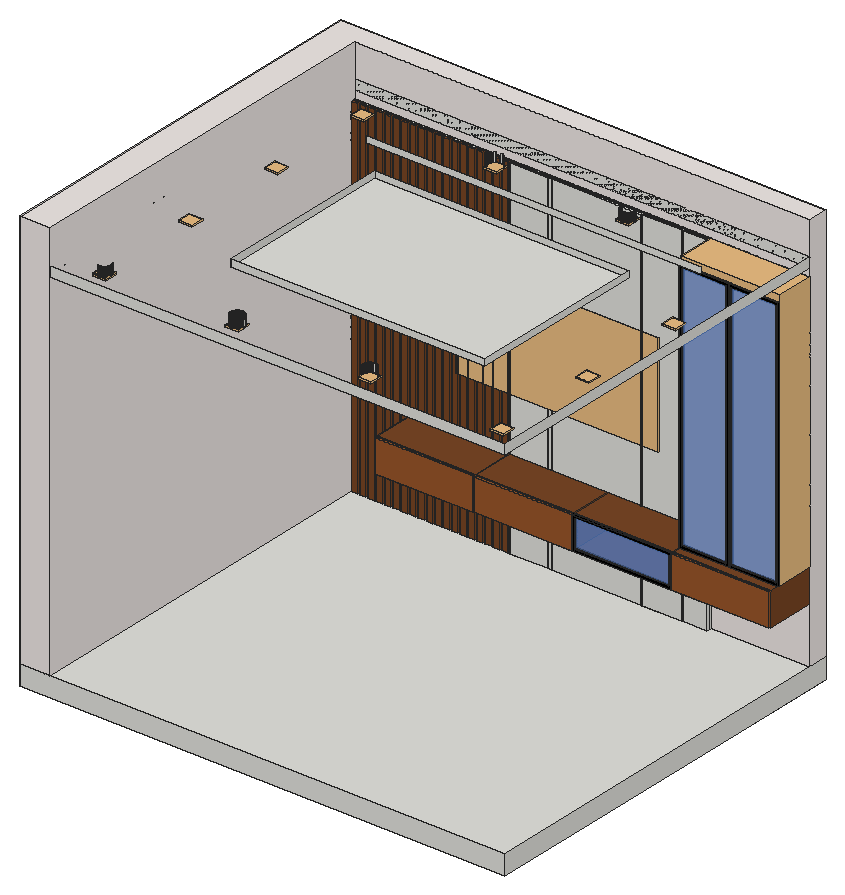
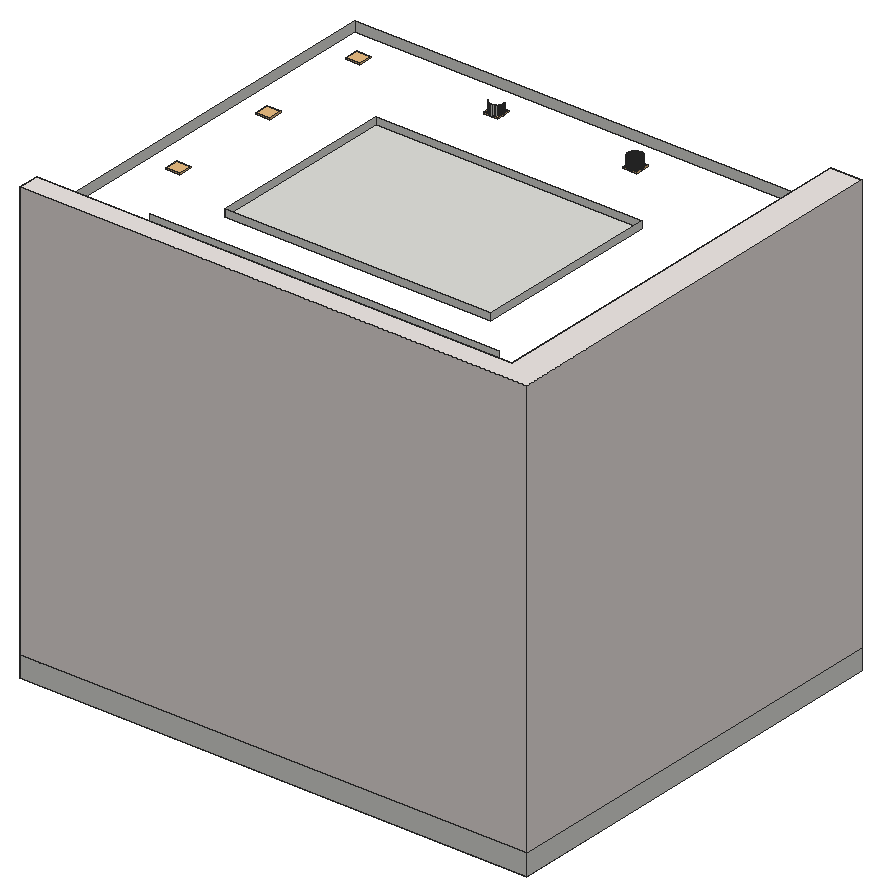
# SketchUp Ruby script. Lengths in millimetres.
U = 1.mm
M = Sketchup.active_model
def pt(a) = Geom::Point3d.new(a.map { |v| v * U })
def face(e, loops, mat)
  f = e.add_face(loops[0].map { |a| pt(a) })
  loops[1..].each { |l| e.add_face(l.map { |a| pt(a) }).erase! }
  f.material = f.back_material = mat if mat
  f
end
# faces: each face lists its corners as indices into pts; further lists are holes
def faces(e, pts, list, mat = nil) = list.each { |f| face(e, (f[0].is_a?(Array) ? f : [f]).map { |l| l.map { |i| pts[i] } }, mat) }
# xy, xz, yz: faces in a plane at the given z, y or x. An outline is a flat list of corners, or four numbers for a rectangle; further outlines are holes
def ring(l) = l.size == 4 ? [[l[0], l[1]], [l[2], l[1]], [l[2], l[3]], [l[0], l[3]]] : l.each_slice(2).to_a
def flat(e, list, mat, &to3) = list.each { |f| face(e, (f[0].is_a?(Array) ? f : [f]).map { |l| ring(l).map { |u, v| to3.(u, v) } }, mat) }
def xy(e, z, list, mat = nil) = flat(e, list, mat) { |x, y| [x, y, z] }
def xz(e, y, list, mat = nil) = flat(e, list, mat) { |x, z| [x, y, z] }
def yz(e, x, list, mat = nil) = flat(e, list, mat) { |y, z| [x, y, z] }
def lines(e, pts, list) = list.each { |a, b| e.add_line(pt(pts[a]), pt(pts[b])) }
# prism: a flat outline (further loops are holes) pulled along v
def prism(e, loops, v, mat = nil)
  f = face(e, loops, mat); d = Geom::Vector3d.new(v.map { |x| x * U })
  f.pushpull(f.normal.samedirection?(d) ? d.length : -d.length)
end
def box(e, o, s, mat = nil) = prism(e, [[o, [o[0] + s[0], o[1], o[2]], [o[0] + s[0], o[1] + s[1], o[2]], [o[0], o[1] + s[1], o[2]]]], [0, 0, s[2]], mat)
def at(x, y, z, deg = 0) = Geom::Transformation.translation(pt([x, y, z])) * Geom::Transformation.rotation(ORIGIN, Z_AXIS, deg.degrees)
def axes(o, x, y, z) = Geom::Transformation.new([*x, 0, *y, 0, *z, 0, *pt(o).to_a, 1])
def part(name) = M.definitions.add(name)
# library, detail: a bought-in or finely detailed component or shape, given as its bounding box
def library(name, o, s) = part(name).tap { |d| box(d.entities, o, s) }
def detail(e, o, s) = box(e.add_group.entities, o, s)
def put(e, d, t, mat = nil) = e.add_instance(d, t).tap { |i| i.material = mat if mat }
def group(e, t, mat = nil) = e.add_group.tap { |g| g.transformation = t; g.material = mat if mat }.entities
root = M.entities
M.materials.add("0209 AP 9428 SKY PINK").color = [239, 232, 229]
M.materials.add("0235 AP 9121 dancing pink").color = [200, 173, 206]
M.materials.add("[0137_Black]").color = [0, 0, 0]
M.materials.add("[Translucent Glass Blue]").color = [100, 149, 237]
M.materials["[Translucent Glass Blue]"].alpha = 0.5
M.materials.add("[Wood Cherry Original]").color = [152, 86, 42]
M.materials.add("[Wood Veneer 01]").color = [120, 70, 37]
c1 = part("Group\#21")
box(c1.entities,[-2669.7,0,0],[3683.6,3048,150])
c2 = part("WOODEN PANELLING")
box(c2.entities,[0,-18,-2660],[50.8,18,2660],"[Wood Veneer 01]")
c3 = part("Group\#12")
xy(c3.entities,0,[[0,0,750,362]])
xy(c3.entities,18,[[18,0,732,344]])
xy(c3.entities,232,[[18,0,732,344]])
xy(c3.entities,250,[[0,0,750,362]])
xz(c3.entities,0,[[[0,0,750,250],[18,18,732,232]]])
xz(c3.entities,344,[[18,18,732,232]])
xz(c3.entities,362,[[0,0,750,250]])
yz(c3.entities,0,[[0,0,362,250]])
yz(c3.entities,18,[[0,18,344,232]])
yz(c3.entities,732,[[0,18,344,232]])
yz(c3.entities,750,[[0,0,362,250]])
c4 = part("Group\#4")
xy(c4.entities,3,[[3,0,747,18]])
xy(c4.entities,247,[[3,0,747,18]])
xz(c4.entities,0,[[3,3,747,247]])
xz(c4.entities,18,[[[0,0,750,250],[3,3,747,247]]])
yz(c4.entities,3,[[0,3,18,247]])
yz(c4.entities,747,[[0,3,18,247]])
c5 = library("Group\#7",[0,0,0],[750,282,1980])
c6 = library("Television screen",[0,35.9,29],[912.5,6.9,513.2])
c7 = library("Group\#29",[0,0,0],[100,99.8,10])
c8 = library("Group\#23",[0,0,0],[100,99.8,10])
c9 = library("Group\#22",[0,0,0],[100,99.8,10])
c10 = library("Group\#24",[0,0,0],[100,99.8,10])
c11 = library("Group\#25",[0,0,0],[100,99.8,10])
c12 = library("Group\#27",[0,0,0],[100,99.8,10])
c13 = library("Group\#26",[0,0,0],[100,99.8,10])
xy(root,2718.2,[[990.6,762,2921.6,2133.6]])
xz(root,0,[[228.6,2718.2,3683.6,2794]])
xz(root,762,[[990.6,2718.2,2921.6,2768.6]])
xz(root,2133.6,[[990.6,2718.2,2921.6,2768.6]])
xz(root,2438.4,[[685.8,2718.2,3226.4,2766.6]])
xz(root,2895.6,[[228.6,2718.2,3683.6,2794]])
yz(root,228.6,[[0,2718.2,2895.6,2794]])
yz(root,990.6,[[762,2718.2,2133.6,2768.6]])
yz(root,2921.6,[[762,2718.2,2133.6,2768.6]])
yz(root,3683.6,[[0,2718.2,2895.6,2794]])
p = [[457.2,177.8,2794],[457.2,177.8,2718.2],[454,177.9,2718.2],[454,177.9,2794],[460.4,177.9,2794],[460.4,177.9,2718.2],
  [1465.5,177.8,2794],[1465.5,177.8,2718.2],[1462.3,177.9,2718.2],[1462.3,177.9,2794],[1468.7,177.9,2794],[1468.7,177.9,2718.2],
  [450.8,178.2,2718.2],[450.8,178.2,2794],[463.6,178.2,2794],[463.6,178.2,2718.2],[1459.2,178.2,2718.2],[1459.2,178.2,2794],
  [1471.9,178.2,2794],[1471.9,178.2,2718.2],[447.7,178.7,2718.2],[447.7,178.7,2794],[466.7,178.7,2794],[466.7,178.7,2718.2],
  [1456,178.7,2718.2],[1456,178.7,2794],[1475.1,178.7,2794],[1475.1,178.7,2718.2],[444.6,179.4,2718.2],[444.6,179.4,2794],
  [469.8,179.4,2794],[469.8,179.4,2718.2],[1452.9,179.4,2718.2],[1452.9,179.4,2794],[1478.2,179.4,2794],[1478.2,179.4,2718.2],
  [472.9,180.3,2794],[472.9,180.3,2718.2],[1449.8,180.3,2718.2],[1449.8,180.3,2794],[1481.2,180.3,2794],[1481.2,180.3,2718.2],
  [475.9,181.4,2794],[475.9,181.4,2718.2],[1446.8,181.4,2718.2],[1446.8,181.4,2794],[1484.2,181.4,2794],[1484.2,181.4,2718.2],
  [478.8,182.6,2794],[478.8,182.6,2718.2],[1443.9,182.6,2718.2],[1443.9,182.6,2794],[1487.2,182.6,2794],[1487.2,182.6,2718.2],
  [481.7,184.1,2794],[481.7,184.1,2718.2],[1441.1,184.1,2718.2],[1441.1,184.1,2794],[1490,184.1,2794],[1490,184.1,2718.2],
  [484.4,185.7,2794],[484.4,185.7,2718.2],[1438.3,185.7,2718.2],[1438.3,185.7,2794],[1492.8,185.7,2794],[1492.8,185.7,2718.2],
  [487.1,187.5,2794],[487.1,187.5,2718.2],[1435.7,187.5,2718.2],[1435.7,187.5,2794],[1495.4,187.5,2794],[1495.4,187.5,2718.2],
  [489.6,189.5,2794],[489.6,189.5,2718.2],[1433.2,189.5,2718.2],[1433.2,189.5,2794],[1497.9,189.5,2794],[1497.9,189.5,2718.2],
  [492,191.6,2794],[492,191.6,2718.2],[1430.8,191.6,2718.2],[1430.8,191.6,2794],[1500.3,191.6,2794],[1500.3,191.6,2718.2],
  [494.2,193.8,2794],[494.2,193.8,2718.2],[1428.5,193.8,2718.2],[1428.5,193.8,2794],[1502.6,193.8,2794],[1502.6,193.8,2718.2],
  [496.3,196.2,2794],[496.3,196.2,2718.2],[1426.4,196.2,2718.2],[1426.4,196.2,2794],[1504.7,196.2,2794],[1504.7,196.2,2718.2],
  [498.3,198.7,2794],[498.3,198.7,2718.2],[1424.4,198.7,2718.2],[1424.4,198.7,2794],[1506.6,198.7,2794],[1506.6,198.7,2718.2],
  [500.1,201.4,2794],[500.1,201.4,2718.2],[1422.6,201.4,2718.2],[1422.6,201.4,2794],[1508.4,201.4,2794],[1508.4,201.4,2718.2],
  [501.7,204.1,2794],[501.7,204.1,2718.2],[1421,204.1,2718.2],[1421,204.1,2794],[1510,204.1,2794],[1510,204.1,2718.2],
  [503.2,207,2794],[503.2,207,2718.2],[1419.6,207,2718.2],[1419.6,207,2794],[1511.5,207,2794],[1511.5,207,2718.2],
  [504.4,209.9,2794],[504.4,209.9,2718.2],[1418.3,209.9,2718.2],[1418.3,209.9,2794],[1512.8,209.9,2794],[1512.8,209.9,2718.2],
  [505.5,212.9,2794],[505.5,212.9,2718.2],[1417.2,212.9,2718.2],[1417.2,212.9,2794],[1513.8,212.9,2794],[1513.8,212.9,2718.2],
  [506.4,216,2794],[506.4,216,2718.2],[1416.3,216,2718.2],[1416.3,216,2794],[1514.7,216,2794],[1514.7,216,2718.2],
  [2425.6,212.9,2794],[2425.6,212.9,2718.2],[2424.7,216,2718.2],[2424.7,216,2794],[507.1,219.1,2794],[507.1,219.1,2718.2],
  [1415.6,219.1,2718.2],[1415.6,219.1,2794],[1515.4,219.1,2794],[1515.4,219.1,2718.2],[2424,219.1,2718.2],[2424,219.1,2794],
  [507.6,222.2,2794],[507.6,222.2,2718.2],[1415.1,222.2,2718.2],[1415.1,222.2,2794],[1515.9,222.2,2794],[1515.9,222.2,2718.2],
  [2423.5,222.2,2718.2],[2423.5,222.2,2794],[507.9,225.4,2794],[507.9,225.4,2718.2],[1414.8,225.4,2718.2],[1414.8,225.4,2794],
  [2423.2,225.4,2718.2],[2423.2,225.4,2794],[508,228.6,2794],[508,228.6,2718.2],[1414.7,228.6,2718.2],[1414.7,228.6,2794],
  [1516.3,228.6,2794],[1516.3,228.6,2718.2],[1516.2,225.4,2718.2],[1516.2,225.4,2794],[2423.1,228.6,2718.2],[2423.1,228.6,2794],
  [507.9,231.8,2794],[507.9,231.8,2718.2],[1414.8,231.8,2718.2],[1414.8,231.8,2794],[1516.2,231.8,2794],[1516.2,231.8,2718.2],
  [2423.2,231.8,2718.2],[2423.2,231.8,2794],[507.6,235,2794],[507.6,235,2718.2],[1415.1,235,2718.2],[1415.1,235,2794],
  [1515.9,235,2794],[1515.9,235,2718.2],[507.1,238.1,2794],[507.1,238.1,2718.2],[1415.6,238.1,2718.2],[1415.6,238.1,2794],
  [1515.4,238.1,2794],[1515.4,238.1,2718.2],[506.4,241.2,2794],[506.4,241.2,2718.2],[1416.3,241.2,2718.2],[1416.3,241.2,2794],
  [505.5,244.3,2794],[505.5,244.3,2718.2],[1417.2,244.3,2718.2],[1417.2,244.3,2794],[2424.7,241.2,2794],[2424.7,241.2,2718.2],
  [2425.6,244.3,2718.2],[2425.6,244.3,2794],[504.4,247.3,2794],[504.4,247.3,2718.2],[1418.3,247.3,2718.2],[1418.3,247.3,2794],
  [2426.6,247.3,2718.2],[2426.6,247.3,2794],[503.2,250.2,2794],[503.2,250.2,2718.2],[1419.6,250.2,2718.2],[1419.6,250.2,2794],
  [501.7,253.1,2794],[501.7,253.1,2718.2],[1421,253.1,2718.2],[1421,253.1,2794],[1510,253.1,2794],[1510,253.1,2718.2],
  [1511.5,250.2,2718.2],[1511.5,250.2,2794],[2427.9,250.2,2794],[2427.9,250.2,2718.2],[2429.4,253.1,2718.2],[2429.4,253.1,2794],
  [1422.6,255.8,2718.2],[1422.6,255.8,2794],[1508.4,255.8,2794],[1508.4,255.8,2718.2],[2431,255.8,2718.2],[2431,255.8,2794],
  [2516.8,255.8,2794],[2516.8,255.8,2718.2],[2518.4,253.1,2718.2],[2518.4,253.1,2794],[1424.4,258.5,2718.2],[1424.4,258.5,2794],
  [1506.6,258.5,2794],[1506.6,258.5,2718.2],[2432.8,258.5,2718.2],[2432.8,258.5,2794],[2515,258.5,2794],[2515,258.5,2718.2],
  [1426.4,261,2718.2],[1426.4,261,2794],[1504.7,261,2794],[1504.7,261,2718.2],[2513,261,2794],[2513,261,2718.2],
  [1428.5,263.4,2718.2],[1428.5,263.4,2794],[1502.6,263.4,2794],[1502.6,263.4,2718.2],[2510.9,263.4,2794],[2510.9,263.4,2718.2],
  [1430.8,265.6,2718.2],[1430.8,265.6,2794],[1500.3,265.6,2794],[1500.3,265.6,2718.2],[2508.6,265.6,2794],[2508.6,265.6,2718.2],
  [1433.2,267.7,2718.2],[1433.2,267.7,2794],[1497.9,267.7,2794],[1497.9,267.7,2718.2],[1435.7,269.7,2718.2],[1435.7,269.7,2794],
  [1495.4,269.7,2794],[1495.4,269.7,2718.2],[2441.5,267.7,2794],[2441.5,267.7,2718.2],[2444,269.7,2718.2],[2444,269.7,2794],
  [2503.7,269.7,2794],[2503.7,269.7,2718.2],[2506.2,267.7,2718.2],[2506.2,267.7,2794],[1438.3,271.5,2718.2],[1438.3,271.5,2794],
  [1492.8,271.5,2794],[1492.8,271.5,2718.2],[2446.6,271.5,2718.2],[2446.6,271.5,2794],[2501.1,271.5,2794],[2501.1,271.5,2718.2],
  [1441.1,273.1,2718.2],[1441.1,273.1,2794],[1490,273.1,2794],[1490,273.1,2718.2],[2449.4,273.1,2718.2],[2449.4,273.1,2794],
  [2498.3,273.1,2794],[2498.3,273.1,2718.2],[1443.9,274.6,2718.2],[1443.9,274.6,2794],[1487.2,274.6,2794],[1487.2,274.6,2718.2],
  [2452.2,274.6,2718.2],[2452.2,274.6,2794],[2495.5,274.6,2794],[2495.5,274.6,2718.2],[1446.8,275.8,2718.2],[1446.8,275.8,2794],
  [1484.2,275.8,2794],[1484.2,275.8,2718.2],[2492.6,275.8,2794],[2492.6,275.8,2718.2],[1449.8,276.9,2718.2],[1449.8,276.9,2794],
  [1481.2,276.9,2794],[1481.2,276.9,2718.2],[2455.2,275.8,2794],[2455.2,275.8,2718.2],[2458.2,276.9,2718.2],[2458.2,276.9,2794],
  [1452.9,277.8,2718.2],[1452.9,277.8,2794],[1478.2,277.8,2794],[1478.2,277.8,2718.2],[2461.2,277.8,2718.2],[2461.2,277.8,2794],
  [2486.5,277.8,2794],[2486.5,277.8,2718.2],[2489.6,276.9,2718.2],[2489.6,276.9,2794],[1456,278.5,2718.2],[1456,278.5,2794],
  [1475.1,278.5,2794],[1475.1,278.5,2718.2],[2483.4,278.5,2794],[2483.4,278.5,2718.2],[1459.2,279,2718.2],[1459.2,279,2794],
  [1471.9,279,2794],[1471.9,279,2718.2],[2480.2,279,2794],[2480.2,279,2718.2],[1462.3,279.3,2718.2],[1462.3,279.3,2794],
  [1468.7,279.3,2794],[1468.7,279.3,2718.2],[2467.5,279,2794],[2467.5,279,2718.2],[2470.7,279.3,2718.2],[2470.7,279.3,2794],
  [2477.1,279.3,2794],[2477.1,279.3,2718.2],[1465.5,279.4,2718.2],[1465.5,279.4,2794],[2473.9,279.4,2718.2],[2473.9,279.4,2794],
  [2470.7,2630.9,2718.2],[2470.7,2630.9,2794],[2473.9,2630.8,2794],[2473.9,2630.8,2718.2],[2477.1,2630.9,2794],[2477.1,2630.9,2718.2],
  [2467.5,2631.2,2718.2],[2467.5,2631.2,2794],[2480.2,2631.2,2794],[2480.2,2631.2,2718.2],[2464.3,2631.7,2718.2],[2464.3,2631.7,2794],
  [2483.4,2631.7,2794],[2483.4,2631.7,2718.2],[2461.2,2632.4,2718.2],[2461.2,2632.4,2794],[2486.5,2632.4,2794],[2486.5,2632.4,2718.2],
  [2458.2,2633.3,2718.2],[2458.2,2633.3,2794],[2489.6,2633.3,2794],[2489.6,2633.3,2718.2],[2455.2,2634.4,2718.2],[2455.2,2634.4,2794],
  [2492.6,2634.4,2794],[2492.6,2634.4,2718.2],[2452.2,2635.6,2718.2],[2452.2,2635.6,2794],[2495.5,2635.6,2794],[2495.5,2635.6,2718.2],
  [2449.4,2637.1,2718.2],[2449.4,2637.1,2794],[2498.3,2637.1,2794],[2498.3,2637.1,2718.2],[2446.6,2638.7,2718.2],[2446.6,2638.7,2794],
  [2501.1,2638.7,2794],[2501.1,2638.7,2718.2],[2444,2640.5,2718.2],[2444,2640.5,2794],[2503.7,2640.5,2794],[2503.7,2640.5,2718.2],
  [2441.5,2642.5,2718.2],[2441.5,2642.5,2794],[2506.2,2642.5,2794],[2506.2,2642.5,2718.2],[2439.1,2644.6,2718.2],[2439.1,2644.6,2794],
  [2508.6,2644.6,2794],[2508.6,2644.6,2718.2],[1428.5,2646.8,2718.2],[1428.5,2646.8,2794],[1430.8,2644.6,2794],[1430.8,2644.6,2718.2],
  [2436.8,2646.8,2718.2],[2436.8,2646.8,2794],[2510.9,2646.8,2794],[2510.9,2646.8,2718.2],[1426.4,2649.2,2718.2],[1426.4,2649.2,2794],
  [2434.7,2649.2,2718.2],[2434.7,2649.2,2794],[2513,2649.2,2794],[2513,2649.2,2718.2],[1424.4,2651.7,2718.2],[1424.4,2651.7,2794],
  [2432.8,2651.7,2718.2],[2432.8,2651.7,2794],[2515,2651.7,2794],[2515,2651.7,2718.2],[1422.6,2654.4,2718.2],[1422.6,2654.4,2794],
  [2431,2654.4,2718.2],[2431,2654.4,2794],[2516.8,2654.4,2794],[2516.8,2654.4,2718.2],[1421,2657.1,2718.2],[1421,2657.1,2794],
  [2429.4,2657.1,2718.2],[2429.4,2657.1,2794],[2518.4,2657.1,2794],[2518.4,2657.1,2718.2],[1419.6,2660,2718.2],[1419.6,2660,2794],
  [2427.9,2660,2718.2],[2427.9,2660,2794],[2519.8,2660,2794],[2519.8,2660,2718.2],[2426.6,2662.9,2718.2],[2426.6,2662.9,2794],
  [2521.1,2662.9,2794],[2521.1,2662.9,2718.2],[1417.2,2665.9,2718.2],[1417.2,2665.9,2794],[1418.3,2662.9,2794],[1418.3,2662.9,2718.2],
  [2425.6,2665.9,2718.2],[2425.6,2665.9,2794],[2522.2,2665.9,2794],[2522.2,2665.9,2718.2],[1416.3,2669,2718.2],[1416.3,2669,2794],
  [2424.7,2669,2718.2],[2424.7,2669,2794],[2523.1,2669,2794],[2523.1,2669,2718.2],[2424,2672.1,2718.2],[2424,2672.1,2794],
  [2523.8,2672.1,2794],[2523.8,2672.1,2718.2],[2423.5,2675.2,2718.2],[2423.5,2675.2,2794],[2524.3,2675.2,2794],[2524.3,2675.2,2718.2],
  [2423.2,2678.4,2718.2],[2423.2,2678.4,2794],[2524.6,2678.4,2794],[2524.6,2678.4,2718.2],[2423.1,2681.6,2718.2],[2423.1,2681.6,2794],
  [2524.7,2681.6,2794],[2524.7,2681.6,2718.2],[2423.2,2684.8,2718.2],[2423.2,2684.8,2794],[2524.6,2684.8,2794],[2524.6,2684.8,2718.2],
  [2423.5,2688,2718.2],[2423.5,2688,2794],[2524.3,2688,2794],[2524.3,2688,2718.2],[2523.8,2691.1,2794],[2523.8,2691.1,2718.2],
  [1416.3,2694.2,2718.2],[1416.3,2694.2,2794],[1415.6,2691.1,2794],[1415.6,2691.1,2718.2],[2523.1,2694.2,2794],[2523.1,2694.2,2718.2],
  [1417.2,2697.3,2718.2],[1417.2,2697.3,2794],[2522.2,2697.3,2794],[2522.2,2697.3,2718.2],[1418.3,2700.3,2718.2],[1418.3,2700.3,2794],
  [2521.1,2700.3,2794],[2521.1,2700.3,2718.2],[1419.6,2703.2,2718.2],[1419.6,2703.2,2794],[2519.8,2703.2,2794],[2519.8,2703.2,2718.2],
  [1421,2706.1,2718.2],[1421,2706.1,2794],[2518.4,2706.1,2794],[2518.4,2706.1,2718.2],[1510,2706.1,2718.2],[1510,2706.1,2794],
  [1508.4,2708.8,2794],[1508.4,2708.8,2718.2],[1506.6,2711.5,2794],[1506.6,2711.5,2718.2],[1504.7,2714,2794],[1504.7,2714,2718.2],
  [1502.6,2716.4,2794],[1502.6,2716.4,2718.2],[1430.8,2718.6,2718.2],[1430.8,2718.6,2794],[1428.5,2716.4,2794],[1428.5,2716.4,2718.2],
  [1500.3,2718.6,2794],[1500.3,2718.6,2718.2],[1433.2,2720.7,2718.2],[1433.2,2720.7,2794],[1435.7,2722.7,2718.2],[1435.7,2722.7,2794],
  [1490,2726.1,2718.2],[1490,2726.1,2794],[1487.2,2727.6,2794],[1487.2,2727.6,2718.2],[1484.2,2728.8,2794],[1484.2,2728.8,2718.2],
  [1481.2,2729.9,2718.2],[1481.2,2729.9,2794],[1478.2,2730.8,2794],[1478.2,2730.8,2718.2],[1475.1,2731.5,2794],[1475.1,2731.5,2718.2],
  [1471.9,2732,2794],[1471.9,2732,2718.2]]
faces(root,p,[[0,1,2,3],[4,5,1,0],[6,7,8,9],[10,11,7,6],[3,2,12,13],[14,15,5,4],[9,8,16,17],[18,19,11,10],
  [13,12,20,21],[22,23,15,14],[17,16,24,25],[26,27,19,18],[21,20,28,29],[30,31,23,22],[25,24,32,33],[34,35,27,26],
  [36,37,31,30],[33,32,38,39],[40,41,35,34],[42,43,37,36],[39,38,44,45],[46,47,41,40],[48,49,43,42],[45,44,50,51],
  [52,53,47,46],[54,55,49,48],[51,50,56,57],[58,59,53,52],[60,61,55,54],[57,56,62,63],[64,65,59,58],[66,67,61,60],
  [63,62,68,69],[70,71,65,64],[72,73,67,66],[69,68,74,75],[76,77,71,70],[78,79,73,72],[75,74,80,81],[82,83,77,76],
  [84,85,79,78],[81,80,86,87],[88,89,83,82],[90,91,85,84],[87,86,92,93],[94,95,89,88],[96,97,91,90],[93,92,98,99],
  [100,101,95,94],[102,103,97,96],[99,98,104,105],[106,107,101,100],[108,109,103,102],[105,104,110,111],[112,113,107,106],[114,115,109,108],
  [111,110,116,117],[118,119,113,112],[120,121,115,114],[117,116,122,123],[124,125,119,118],[126,127,121,120],[123,122,128,129],[130,131,125,124],
  [132,133,127,126],[129,128,134,135],[136,137,131,130],[138,139,140,141],[142,143,133,132],[135,134,144,145],[146,147,137,136],[141,140,148,149],
  [150,151,143,142],[145,144,152,153],[154,155,147,146],[149,148,156,157],[158,159,151,150],[153,152,160,161],[157,156,162,163],[164,165,159,158],
  [161,160,166,167],[168,169,170,171],[163,162,172,173],[174,175,165,164],[167,166,176,177],[178,179,169,168],[173,172,180,181],[182,183,175,174],
  [177,176,184,185],[186,187,179,178],[188,189,183,182],[185,184,190,191],[192,193,187,186],[194,195,189,188],[191,190,196,197],[198,199,195,194],
  [197,196,200,201],[202,203,204,205],[206,207,199,198],[201,200,208,209],[205,204,210,211],[212,213,207,206],[209,208,214,215],[216,217,213,212],
  [215,214,218,219],[220,221,222,223],[224,225,226,227],[219,218,228,229],[230,231,221,220],[227,226,232,233],[234,235,236,237],[229,228,238,239],
  [240,241,231,230],[233,232,242,243],[244,245,235,234],[239,238,246,247],[248,249,241,240],[250,251,245,244],[247,246,252,253],[254,255,249,248],
  [256,257,251,250],[253,252,258,259],[260,261,255,254],[262,263,257,256],[259,258,264,265],[266,267,261,260],[265,264,268,269],[270,271,267,266],
  [272,273,274,275],[276,277,278,279],[269,268,280,281],[282,283,271,270],[275,274,284,285],[286,287,277,276],[281,280,288,289],[290,291,283,282],
  [285,284,292,293],[294,295,287,286],[289,288,296,297],[298,299,291,290],[293,292,300,301],[302,303,295,294],[297,296,304,305],[306,307,299,298],
  [308,309,303,302],[305,304,310,311],[312,313,307,306],[314,315,316,317],[311,310,318,319],[320,321,313,312],[317,316,322,323],[324,325,326,327],
  [319,318,328,329],[330,331,321,320],[332,333,325,324],[329,328,334,335],[336,337,331,330],[338,339,333,332],[335,334,340,341],[342,343,337,336],
  [344,345,346,347],[348,349,339,338],[341,340,350,351],[351,350,343,342],[347,346,352,353],[354,355,356,357],[357,356,358,359],[360,361,355,354],
  [359,358,362,363],[364,365,361,360],[363,362,366,367],[368,369,365,364],[367,366,370,371],[372,373,369,368],[371,370,374,375],[376,377,373,372],
  [375,374,378,379],[380,381,377,376],[379,378,382,383],[384,385,381,380],[383,382,386,387],[388,389,385,384],[387,386,390,391],[392,393,389,388],
  [391,390,394,395],[396,397,393,392],[395,394,398,399],[400,401,397,396],[399,398,402,403],[404,405,406,407],[408,409,401,400],[403,402,410,411],
  [412,413,405,404],[414,415,409,408],[411,410,416,417],[418,419,413,412],[420,421,415,414],[417,416,422,423],[424,425,419,418],[426,427,421,420],
  [423,422,428,429],[430,431,425,424],[432,433,427,426],[429,428,434,435],[436,437,431,430],[438,439,433,432],[435,434,440,441],[442,443,439,438],
  [441,440,444,445],[446,447,448,449],[450,451,443,442],[445,444,452,453],[454,455,447,446],[456,457,451,450],[453,452,458,459],[460,461,457,456],
  [459,458,462,463],[464,465,461,460],[463,462,466,467],[468,469,465,464],[467,466,470,471],[472,473,469,468],[471,470,474,475],[476,477,473,472],
  [475,474,478,479],[480,481,477,476],[479,478,482,483],[483,482,484,485],[486,487,488,489],[485,484,490,491],[492,493,487,486],[491,490,494,495],
  [496,497,493,492],[495,494,498,499],[500,501,497,496],[499,498,502,503],[504,505,501,500],[503,502,506,507],[508,509,510,511],[511,510,512,513],
  [513,512,514,515],[515,514,516,517],[518,519,520,521],[517,516,522,523],[524,525,519,518],[526,527,525,524],[528,529,530,531],[531,530,532,533],
  [534,535,536,537],[537,536,538,539],[539,538,540,541]])
put(root,c1,at(2669.7,0,-150))
g1 = group(root,at(0,2438.4,0),"0235 AP 9121 dancing pink")
prism(g1,[[[0,609.6,0],[3683.6,609.6,0],[3683.6,457.2,0],[228.6,457.2,0],[228.6,-2438.4,0],[0,-2438.4,0]]],[0,0,3048],"0209 AP 9428 SKY PINK")
g2 = group(root,at(228.6,2877.6,0))
box(g2,[0,0,0],[2705,18,2660])
put(g2,c2,at(0,0,2660))
put(g2,c2,at(63.5,0,2660))
put(g2,c2,at(127,0,2660))
put(g2,c2,at(190.5,0,2660))
put(g2,c2,at(254,0,2660))
put(g2,c2,at(317.5,0,2660))
put(g2,c2,at(381,0,2660))
put(g2,c2,at(444.5,0,2660))
put(g2,c2,at(508,0,2660))
put(g2,c2,at(571.5,0,2660))
put(g2,c2,at(635,0,2660))
put(g2,c2,at(698.5,0,2660))
put(g2,c2,at(762,0,2660))
put(g2,c2,at(825.5,0,2660))
put(g2,c2,at(889,0,2660))
put(g2,c2,at(952.5,0,2660))
put(g2,c2,at(1016,0,2660))
put(g2,c2,at(1079.5,0,2660))
put(g2,c2,at(1143,0,2660))
g3 = group(root,at(228.6,2859.6,0))
xy(g3,0,[[1200,0,1208,18],[1208,0,1493,18],[1493,0,1523,18],[1523,0,2204,18],[2204,0,2212,18],
  [2212,0,2513,18],[2513,0,2521,18],[2521,0,2705,18]])
xy(g3,2660,[[1200,0,1208,18],[1208,0,1493,18],[1493,0,1523,18],[1523,0,2204,18],[2204,0,2212,18],
  [2212,0,2513,18],[2513,0,2521,18],[2521,0,2705,18]])
xz(g3,0,[[1200,0,1208,2660],[1208,0,1493,2660],[1493,0,1523,2660],[1523,0,2204,2660],[2204,0,2212,2660],
  [2212,0,2513,2660],[2513,0,2521,2660],[2521,0,2705,2660]])
xz(g3,18,[[1208,0,1493,2660],[1493,0,1523,2660],[1523,0,2204,2660],[2204,0,2212,2660],[2212,0,2513,2660],
  [2513,0,2521,2660],[2521,0,2705,2660]])
yz(g3,1200,[[0,0,18,2660]])
yz(g3,1208,[[0,0,18,2660]])
yz(g3,1493,[[0,0,18,2660]])
yz(g3,1523,[[0,0,18,2660]])
yz(g3,2204,[[0,0,18,2660]])
yz(g3,2212,[[0,0,18,2660]])
yz(g3,2513,[[0,0,18,2660]])
yz(g3,2521,[[0,0,18,2660]])
yz(g3,2705,[[0,0,18,2660]])
put(root,c3,at(683.6,2533.6,430),"[Wood Veneer 01]")
put(root,c4,at(683.6,2515.6,430),"[Wood Cherry Original]")
g4 = group(root,at(1433.6,2533.6,430),"[Wood Veneer 01]")
xy(g4,0,[[0,0,750,362]])
xy(g4,18,[[18,0,732,344]])
xy(g4,232,[[18,0,732,344]])
xy(g4,250,[[0,0,750,362]])
xz(g4,0,[[[0,0,750,250],[18,18,732,232]]])
xz(g4,344,[[18,18,732,232]])
xz(g4,362,[[0,0,750,250]])
yz(g4,0,[[0,0,362,250]])
yz(g4,18,[[0,18,344,232]])
yz(g4,732,[[0,18,344,232]])
yz(g4,750,[[0,0,362,250]])
put(root,c4,at(1433.6,2515.6,430),"[Wood Cherry Original]")
put(root,c3,at(2183.6,2533.6,430),"[Wood Veneer 01]")
put(root,c3,at(2933.6,2533.6,430),"[Wood Veneer 01]")
put(root,c4,at(2933.6,2515.6,430),"[Wood Cherry Original]")
g5 = group(root,at(2183.6,2533.6,430),"[0137_Black]")
prism(g5,[[[0,0,0],[0,0,250],[750,0,250],[750,0,0]],[[18,0,18],[732,0,18],[732,0,232],[18,0,232]]],[0,-18,0])
g6 = group(root,at(2201.6,2533.6,448),"[Translucent Glass Blue]")
box(g6,[0,-5,0],[714,5,214])
g7 = group(root,at(2933.6,2595.6,680),"[0137_Black]")
prism(g7,[[[0,18,0],[0,18,1930],[375,18,1930],[375,18,0]],[[18,18,18],[357,18,18],[357,18,1912],[18,18,1912]]],[0,-18,0])
g8 = group(root,at(3308.6,2595.6,680),"[0137_Black]")
prism(g8,[[[375,18,1930],[375,18,0],[0,18,0],[0,18,1930]],[[18,18,18],[357,18,18],[357,18,1912],[18,18,1912]]],[0,-18,0])
put(root,c5,at(2933.6,2613.6,680),"[Wood Cherry Original]")
g9 = group(root,at(2951.6,2613.6,698),"[Translucent Glass Blue]")
box(g9,[0,-9,0],[339,9,1894])
g10 = group(root,at(3326.6,2613.6,698),"[Translucent Glass Blue]")
box(g10,[0,-9,0],[339,9,1894])
put(root,c6,axes([1032.9,2816.8,1047.9],[1.6819,0,0],[0,1,0],[0,0,1.51307]))
put(root,c7,at(407.8,178,2708.2))
put(root,c8,axes([406.3,178,2716.2],[1.01521,0,0],[0,1,0],[0,0,1]))
put(root,c9,axes([3431,178,2716.2],[1.01521,0,0],[0,1,0],[0,0,1]))
put(root,c10,axes([1414.5,178,2716.2],[1.01521,0,0],[0,1,0],[0,0,1]))
put(root,c11,axes([2422.7,178,2716.2],[1.01521,0,0],[0,1,0],[0,0,1]))
put(root,c12,axes([2422.7,2630.3,2716.2],[1.01521,0,0],[0,1,0],[0,0,1]))
put(root,c10,axes([1414.5,2630.3,2716.2],[1.01521,0,0],[0,1,0],[0,0,1]))
put(root,c8,axes([406.3,2630.3,2716.2],[1.01521,0,0],[0,1,0],[0,0,1]))
put(root,c13,axes([3431,992,2716.2],[1.01521,0,0],[0,1,0],[0,0,1]))
put(root,c13,axes([3431,1812,2716.2],[1.01521,0,0],[0,1,0],[0,0,1]))
put(root,c8,axes([406.3,997,2716.2],[1.01521,0,0],[0,1,0],[0,0,1]))
put(root,c8,axes([406.3,1813,2716.2],[1.01521,0,0],[0,1,0],[0,0,1]))
